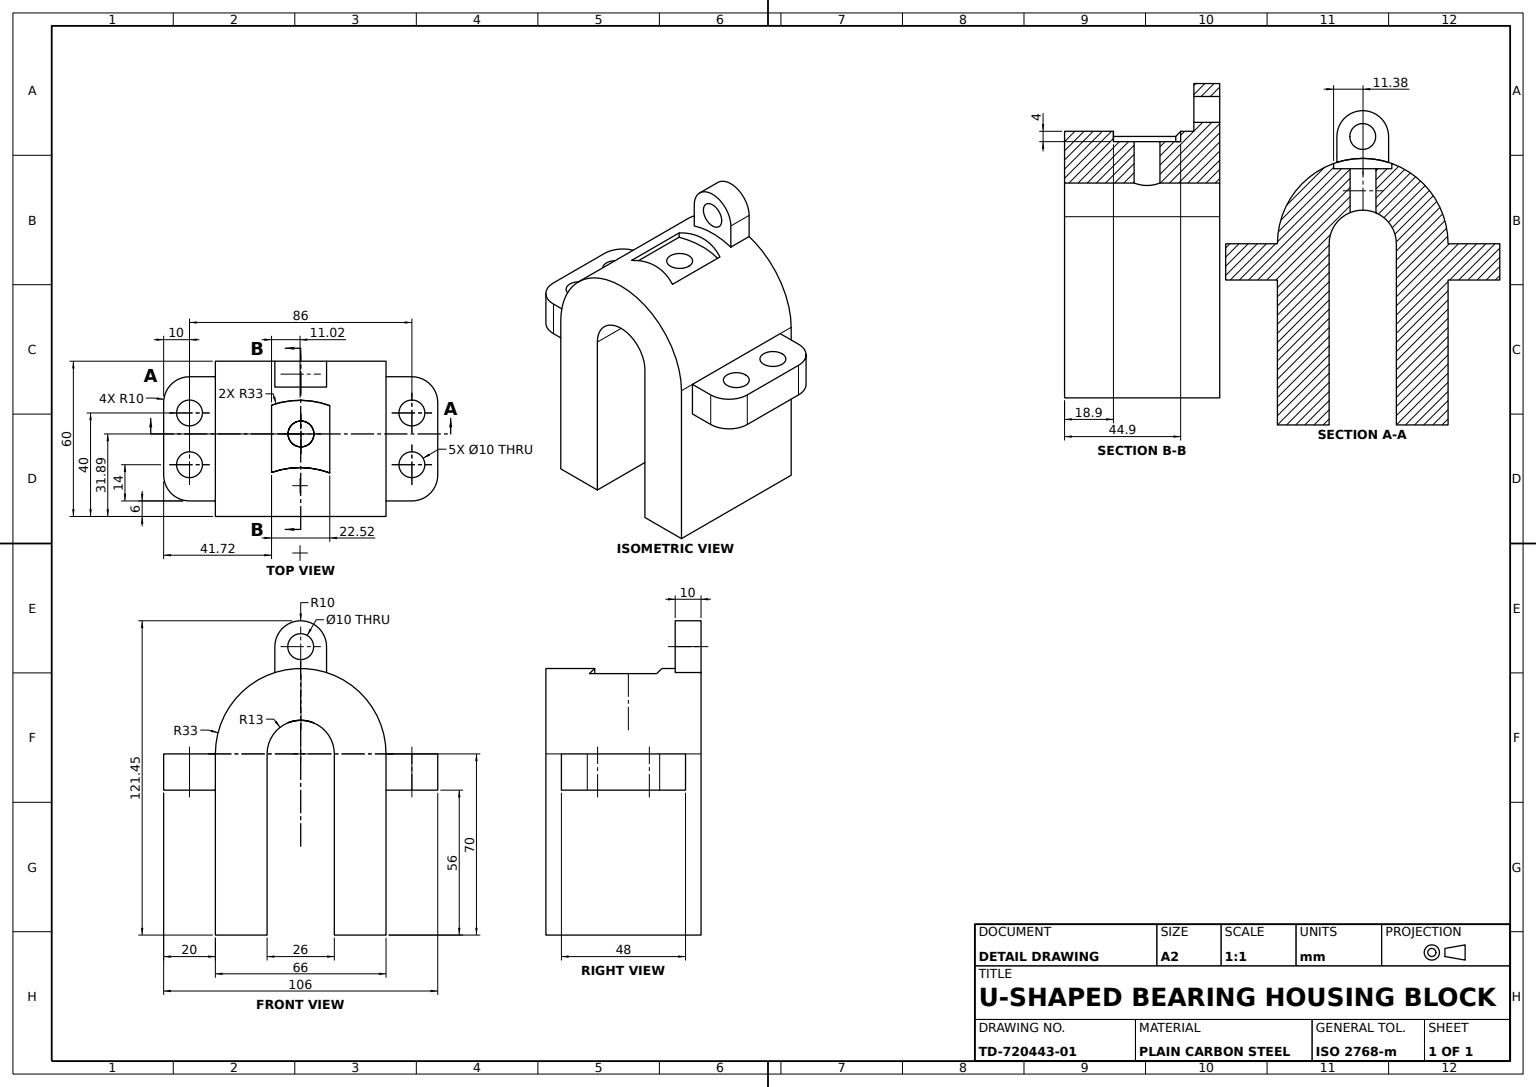
ISO-10303-21;
HEADER;
FILE_DESCRIPTION((''),'2;1');
FILE_NAME('','',(''),(''),'','','');
FILE_SCHEMA(('AUTOMOTIVE_DESIGN'));
ENDSEC;
DATA;
#1=APPLICATION_CONTEXT('');
#2=PRODUCT_CONTEXT('',#1,'mechanical');
#3=PRODUCT('','','',(#2));
#4=PRODUCT_DEFINITION_FORMATION('','',#3);
#5=PRODUCT_DEFINITION_CONTEXT('',#1,'design');
#6=PRODUCT_DEFINITION('','',#4,#5);
#7=PRODUCT_DEFINITION_SHAPE('','',#6);
#8=(LENGTH_UNIT()NAMED_UNIT(*)SI_UNIT(.MILLI.,.METRE.));
#9=(NAMED_UNIT(*)PLANE_ANGLE_UNIT()SI_UNIT($,.RADIAN.));
#10=(NAMED_UNIT(*)SI_UNIT($,.STERADIAN.)SOLID_ANGLE_UNIT());
#11=UNCERTAINTY_MEASURE_WITH_UNIT(LENGTH_MEASURE(1.E-05),#8,'distance_accuracy_value','');
#12=(GEOMETRIC_REPRESENTATION_CONTEXT(3)GLOBAL_UNCERTAINTY_ASSIGNED_CONTEXT((#11))GLOBAL_UNIT_ASSIGNED_CONTEXT((#8,#9,#10))REPRESENTATION_CONTEXT('',''));
#13=CARTESIAN_POINT('',(46.,70.,-60.));
#14=VERTEX_POINT('',#13);
#15=CARTESIAN_POINT('',(46.,0.,-60.));
#16=VERTEX_POINT('',#15);
#17=DIRECTION('',(0.,-1.,0.));
#18=VECTOR('',#17,1000.);
#19=LINE('',#13,#18);
#20=EDGE_CURVE('',#14,#16,#19,.T.);
#21=ORIENTED_EDGE('',*,*,#20,.T.);
#22=CARTESIAN_POINT('',(46.,0.,0.));
#23=VERTEX_POINT('',#22);
#24=DIRECTION('',(0.,0.,1.));
#25=VECTOR('',#24,1000.);
#26=LINE('',#15,#25);
#27=EDGE_CURVE('',#16,#23,#26,.T.);
#28=ORIENTED_EDGE('',*,*,#27,.T.);
#29=CARTESIAN_POINT('',(46.,70.,0.));
#30=VERTEX_POINT('',#29);
#31=LINE('',#29,#18);
#32=EDGE_CURVE('',#30,#23,#31,.T.);
#33=ORIENTED_EDGE('',*,*,#32,.F.);
#34=LINE('',#13,#25);
#35=EDGE_CURVE('',#14,#30,#34,.T.);
#36=ORIENTED_EDGE('',*,*,#35,.F.);
#37=EDGE_LOOP('',(#21,#28,#33,#36));
#38=FACE_OUTER_BOUND('',#37,.T.);
#39=DIRECTION('',(-1.,0.,0.));
#40=AXIS2_PLACEMENT_3D('',#13,#39,#17);
#41=PLANE('',#40);
#42=ADVANCED_FACE('',(#38),#41,.T.);
#43=CARTESIAN_POINT('',(-10.,56.,-54.));
#44=VERTEX_POINT('',#43);
#45=CARTESIAN_POINT('',(-10.,70.,-54.));
#46=VERTEX_POINT('',#45);
#47=DIRECTION('',(0.,1.,0.));
#48=VECTOR('',#47,1000.);
#49=LINE('',#43,#48);
#50=EDGE_CURVE('',#44,#46,#49,.T.);
#51=ORIENTED_EDGE('',*,*,#50,.F.);
#52=CARTESIAN_POINT('',(-20.,56.,-44.));
#53=VERTEX_POINT('',#52);
#54=CARTESIAN_POINT('',(-10.,56.,-44.));
#55=DIRECTION('',(0.,0.,-1.));
#56=AXIS2_PLACEMENT_3D('',#54,#17,#55);
#57=CIRCLE('',#56,10.);
#58=EDGE_CURVE('',#53,#44,#57,.T.);
#59=ORIENTED_EDGE('',*,*,#58,.F.);
#60=CARTESIAN_POINT('',(-20.,70.,-44.));
#61=VERTEX_POINT('',#60);
#62=LINE('',#52,#18);
#63=EDGE_CURVE('',#61,#53,#62,.T.);
#64=ORIENTED_EDGE('',*,*,#63,.F.);
#65=CARTESIAN_POINT('',(-10.,70.,-44.));
#66=AXIS2_PLACEMENT_3D('',#65,#47,#55);
#67=CIRCLE('',#66,10.);
#68=EDGE_CURVE('',#46,#61,#67,.T.);
#69=ORIENTED_EDGE('',*,*,#68,.F.);
#70=EDGE_LOOP('',(#51,#59,#64,#69));
#71=FACE_OUTER_BOUND('',#70,.T.);
#72=AXIS2_PLACEMENT_3D('',#54,#47,#24);
#73=CYLINDRICAL_SURFACE('',#72,10.);
#74=ADVANCED_FACE('',(#71),#73,.T.);
#75=CARTESIAN_POINT('',(20.,70.,-60.));
#76=VERTEX_POINT('',#75);
#77=CARTESIAN_POINT('',(33.,70.,-60.));
#78=AXIS2_PLACEMENT_3D('',#77,#55,#39);
#79=CIRCLE('',#78,13.);
#80=EDGE_CURVE('',#76,#14,#79,.T.);
#81=ORIENTED_EDGE('',*,*,#80,.F.);
#82=CARTESIAN_POINT('',(20.,0.,-60.));
#83=VERTEX_POINT('',#82);
#84=LINE('',#82,#48);
#85=EDGE_CURVE('',#83,#76,#84,.T.);
#86=ORIENTED_EDGE('',*,*,#85,.F.);
#87=CARTESIAN_POINT('',(0.,0.,-60.));
#88=VERTEX_POINT('',#87);
#89=DIRECTION('',(1.,0.,0.));
#90=VECTOR('',#89,1000.);
#91=LINE('',#87,#90);
#92=EDGE_CURVE('',#88,#83,#91,.T.);
#93=ORIENTED_EDGE('',*,*,#92,.F.);
#94=CARTESIAN_POINT('',(0.,70.,-60.));
#95=VERTEX_POINT('',#94);
#96=LINE('',#87,#18);
#97=EDGE_CURVE('',#95,#88,#96,.T.);
#98=ORIENTED_EDGE('',*,*,#97,.F.);
#99=CARTESIAN_POINT('',(23.,101.44837,-60.));
#100=VERTEX_POINT('',#99);
#101=AXIS2_PLACEMENT_3D('',#77,#24,#39);
#102=CIRCLE('',#101,33.);
#103=EDGE_CURVE('',#100,#95,#102,.T.);
#104=ORIENTED_EDGE('',*,*,#103,.F.);
#105=CARTESIAN_POINT('',(23.,111.44837,-60.));
#106=VERTEX_POINT('',#105);
#107=LINE('',#105,#48);
#108=EDGE_CURVE('',#100,#106,#107,.T.);
#109=ORIENTED_EDGE('',*,*,#108,.T.);
#110=CARTESIAN_POINT('',(43.,111.44837,-60.));
#111=VERTEX_POINT('',#110);
#112=CARTESIAN_POINT('',(33.,111.44837,-60.));
#113=AXIS2_PLACEMENT_3D('',#112,#55,#89);
#114=CIRCLE('',#113,10.);
#115=EDGE_CURVE('',#106,#111,#114,.T.);
#116=ORIENTED_EDGE('',*,*,#115,.T.);
#117=CARTESIAN_POINT('',(43.,101.44837,-60.));
#118=VERTEX_POINT('',#117);
#119=LINE('',#117,#18);
#120=EDGE_CURVE('',#111,#118,#119,.T.);
#121=ORIENTED_EDGE('',*,*,#120,.T.);
#122=CARTESIAN_POINT('',(66.,70.,-60.));
#123=VERTEX_POINT('',#122);
#124=EDGE_CURVE('',#123,#118,#102,.T.);
#125=ORIENTED_EDGE('',*,*,#124,.F.);
#126=CARTESIAN_POINT('',(66.,0.,-60.));
#127=VERTEX_POINT('',#126);
#128=LINE('',#122,#48);
#129=EDGE_CURVE('',#127,#123,#128,.T.);
#130=ORIENTED_EDGE('',*,*,#129,.F.);
#131=LINE('',#15,#90);
#132=EDGE_CURVE('',#16,#127,#131,.T.);
#133=ORIENTED_EDGE('',*,*,#132,.F.);
#134=ORIENTED_EDGE('',*,*,#20,.F.);
#135=EDGE_LOOP('',(#81,#86,#93,#98,#104,#109,#116,#121,#125,#130,#133,#134));
#136=FACE_OUTER_BOUND('',#135,.T.);
#137=CARTESIAN_POINT('',(28.,111.44837,-60.));
#138=VERTEX_POINT('',#137);
#139=CARTESIAN_POINT('',(38.,111.44837,-60.));
#140=VERTEX_POINT('',#139);
#141=AXIS2_PLACEMENT_3D('',#112,#55,#39);
#142=CIRCLE('',#141,5.);
#143=EDGE_CURVE('',#138,#140,#142,.T.);
#144=ORIENTED_EDGE('',*,*,#143,.F.);
#145=EDGE_CURVE('',#140,#138,#142,.T.);
#146=ORIENTED_EDGE('',*,*,#145,.F.);
#147=EDGE_LOOP('',(#144,#146));
#148=FACE_BOUND('',#147,.T.);
#149=PLANE('',#78);
#150=ADVANCED_FACE('',(#136,#148),#149,.T.);
#151=CARTESIAN_POINT('',(86.,70.,-44.));
#152=VERTEX_POINT('',#151);
#153=CARTESIAN_POINT('',(76.,70.,-54.));
#154=VERTEX_POINT('',#153);
#155=CARTESIAN_POINT('',(76.,70.,-44.));
#156=AXIS2_PLACEMENT_3D('',#155,#47,#24);
#157=CIRCLE('',#156,10.);
#158=EDGE_CURVE('',#152,#154,#157,.T.);
#159=ORIENTED_EDGE('',*,*,#158,.F.);
#160=CARTESIAN_POINT('',(86.,56.,-44.));
#161=VERTEX_POINT('',#160);
#162=LINE('',#160,#48);
#163=EDGE_CURVE('',#161,#152,#162,.T.);
#164=ORIENTED_EDGE('',*,*,#163,.F.);
#165=CARTESIAN_POINT('',(76.,56.,-54.));
#166=VERTEX_POINT('',#165);
#167=CARTESIAN_POINT('',(76.,56.,-44.));
#168=AXIS2_PLACEMENT_3D('',#167,#17,#24);
#169=CIRCLE('',#168,10.);
#170=EDGE_CURVE('',#166,#161,#169,.T.);
#171=ORIENTED_EDGE('',*,*,#170,.F.);
#172=LINE('',#165,#18);
#173=EDGE_CURVE('',#154,#166,#172,.T.);
#174=ORIENTED_EDGE('',*,*,#173,.F.);
#175=EDGE_LOOP('',(#159,#164,#171,#174));
#176=FACE_OUTER_BOUND('',#175,.T.);
#177=AXIS2_PLACEMENT_3D('',#167,#47,#24);
#178=CYLINDRICAL_SURFACE('',#177,10.);
#179=ADVANCED_FACE('',(#176),#178,.T.);
#180=CARTESIAN_POINT('',(44.244993,99.,-42.828348));
#181=VERTEX_POINT('',#180);
#182=CARTESIAN_POINT('',(44.244993,101.024992,-42.828348));
#183=VERTEX_POINT('',#182);
#184=LINE('',#180,#48);
#185=EDGE_CURVE('',#181,#183,#184,.T.);
#186=ORIENTED_EDGE('',*,*,#185,.F.);
#187=CARTESIAN_POINT('',(44.244993,99.,-16.828348));
#188=VERTEX_POINT('',#187);
#189=VECTOR('',#55,1000.);
#190=LINE('',#180,#189);
#191=EDGE_CURVE('',#188,#181,#190,.T.);
#192=ORIENTED_EDGE('',*,*,#191,.F.);
#193=CARTESIAN_POINT('',(44.244993,101.024992,-16.828348));
#194=VERTEX_POINT('',#193);
#195=LINE('',#187,#48);
#196=EDGE_CURVE('',#188,#194,#195,.T.);
#197=ORIENTED_EDGE('',*,*,#196,.T.);
#198=CARTESIAN_POINT('',(44.244993,101.024992,-60.));
#199=LINE('',#198,#189);
#200=EDGE_CURVE('',#194,#183,#199,.T.);
#201=ORIENTED_EDGE('',*,*,#200,.T.);
#202=EDGE_LOOP('',(#186,#192,#197,#201));
#203=FACE_OUTER_BOUND('',#202,.T.);
#204=AXIS2_PLACEMENT_3D('',#180,#89,#55);
#205=PLANE('',#204);
#206=ADVANCED_FACE('',(#203),#205,.F.);
#207=CARTESIAN_POINT('',(43.,111.44837,-50.));
#208=VERTEX_POINT('',#207);
#209=LINE('',#207,#189);
#210=EDGE_CURVE('',#208,#111,#209,.T.);
#211=ORIENTED_EDGE('',*,*,#210,.F.);
#212=CARTESIAN_POINT('',(43.,101.44837,-50.));
#213=VERTEX_POINT('',#212);
#214=LINE('',#212,#18);
#215=EDGE_CURVE('',#208,#213,#214,.T.);
#216=ORIENTED_EDGE('',*,*,#215,.T.);
#217=LINE('',#212,#189);
#218=EDGE_CURVE('',#213,#118,#217,.T.);
#219=ORIENTED_EDGE('',*,*,#218,.T.);
#220=ORIENTED_EDGE('',*,*,#120,.F.);
#221=EDGE_LOOP('',(#211,#216,#219,#220));
#222=FACE_OUTER_BOUND('',#221,.T.);
#223=AXIS2_PLACEMENT_3D('',#212,#89,#55);
#224=PLANE('',#223);
#225=ADVANCED_FACE('',(#222),#224,.T.);
#226=CARTESIAN_POINT('',(-20.,70.,-16.));
#227=VERTEX_POINT('',#226);
#228=CARTESIAN_POINT('',(-20.,70.,-54.));
#229=LINE('',#228,#25);
#230=EDGE_CURVE('',#61,#227,#229,.T.);
#231=ORIENTED_EDGE('',*,*,#230,.F.);
#232=ORIENTED_EDGE('',*,*,#63,.T.);
#233=CARTESIAN_POINT('',(-20.,56.,-16.));
#234=VERTEX_POINT('',#233);
#235=CARTESIAN_POINT('',(-20.,56.,-54.));
#236=LINE('',#235,#25);
#237=EDGE_CURVE('',#53,#234,#236,.T.);
#238=ORIENTED_EDGE('',*,*,#237,.T.);
#239=LINE('',#233,#48);
#240=EDGE_CURVE('',#234,#227,#239,.T.);
#241=ORIENTED_EDGE('',*,*,#240,.T.);
#242=EDGE_LOOP('',(#231,#232,#238,#241));
#243=FACE_OUTER_BOUND('',#242,.T.);
#244=AXIS2_PLACEMENT_3D('',#235,#39,#24);
#245=PLANE('',#244);
#246=ADVANCED_FACE('',(#243),#245,.T.);
#247=CARTESIAN_POINT('',(86.,70.,-16.));
#248=VERTEX_POINT('',#247);
#249=CARTESIAN_POINT('',(86.,56.,-16.));
#250=VERTEX_POINT('',#249);
#251=LINE('',#249,#18);
#252=EDGE_CURVE('',#248,#250,#251,.T.);
#253=ORIENTED_EDGE('',*,*,#252,.T.);
#254=CARTESIAN_POINT('',(86.,56.,-54.));
#255=LINE('',#254,#189);
#256=EDGE_CURVE('',#250,#161,#255,.T.);
#257=ORIENTED_EDGE('',*,*,#256,.T.);
#258=ORIENTED_EDGE('',*,*,#163,.T.);
#259=CARTESIAN_POINT('',(86.,70.,-54.));
#260=LINE('',#259,#189);
#261=EDGE_CURVE('',#248,#152,#260,.T.);
#262=ORIENTED_EDGE('',*,*,#261,.F.);
#263=EDGE_LOOP('',(#253,#257,#258,#262));
#264=FACE_OUTER_BOUND('',#263,.T.);
#265=AXIS2_PLACEMENT_3D('',#254,#89,#55);
#266=PLANE('',#265);
#267=ADVANCED_FACE('',(#264),#266,.T.);
#268=CARTESIAN_POINT('',(0.,56.,-54.));
#269=VERTEX_POINT('',#268);
#270=CARTESIAN_POINT('',(0.,70.,-54.));
#271=VERTEX_POINT('',#270);
#272=LINE('',#268,#48);
#273=EDGE_CURVE('',#269,#271,#272,.T.);
#274=ORIENTED_EDGE('',*,*,#273,.T.);
#275=LINE('',#94,#25);
#276=EDGE_CURVE('',#95,#271,#275,.T.);
#277=ORIENTED_EDGE('',*,*,#276,.F.);
#278=ORIENTED_EDGE('',*,*,#97,.T.);
#279=CARTESIAN_POINT('',(0.,0.,0.));
#280=VERTEX_POINT('',#279);
#281=LINE('',#87,#25);
#282=EDGE_CURVE('',#88,#280,#281,.T.);
#283=ORIENTED_EDGE('',*,*,#282,.T.);
#284=CARTESIAN_POINT('',(0.,70.,0.));
#285=VERTEX_POINT('',#284);
#286=LINE('',#279,#18);
#287=EDGE_CURVE('',#285,#280,#286,.T.);
#288=ORIENTED_EDGE('',*,*,#287,.F.);
#289=CARTESIAN_POINT('',(0.,70.,-6.));
#290=VERTEX_POINT('',#289);
#291=EDGE_CURVE('',#290,#285,#275,.T.);
#292=ORIENTED_EDGE('',*,*,#291,.F.);
#293=CARTESIAN_POINT('',(0.,56.,-6.));
#294=VERTEX_POINT('',#293);
#295=LINE('',#293,#48);
#296=EDGE_CURVE('',#294,#290,#295,.T.);
#297=ORIENTED_EDGE('',*,*,#296,.F.);
#298=LINE('',#268,#189);
#299=EDGE_CURVE('',#294,#269,#298,.T.);
#300=ORIENTED_EDGE('',*,*,#299,.T.);
#301=EDGE_LOOP('',(#274,#277,#278,#283,#288,#292,#297,#300));
#302=FACE_OUTER_BOUND('',#301,.T.);
#303=AXIS2_PLACEMENT_3D('',#87,#39,#24);
#304=PLANE('',#303);
#305=ADVANCED_FACE('',(#302),#304,.T.);
#306=CARTESIAN_POINT('',(38.,111.44837,-50.));
#307=VERTEX_POINT('',#306);
#308=CARTESIAN_POINT('',(28.,111.44837,-50.));
#309=VERTEX_POINT('',#308);
#310=CARTESIAN_POINT('',(33.,111.44837,-50.));
#311=AXIS2_PLACEMENT_3D('',#310,#55,#39);
#312=CIRCLE('',#311,5.);
#313=EDGE_CURVE('',#307,#309,#312,.T.);
#314=ORIENTED_EDGE('',*,*,#313,.F.);
#315=LINE('',#306,#189);
#316=EDGE_CURVE('',#307,#140,#315,.T.);
#317=ORIENTED_EDGE('',*,*,#316,.T.);
#318=ORIENTED_EDGE('',*,*,#145,.T.);
#319=LINE('',#308,#189);
#320=EDGE_CURVE('',#309,#138,#319,.T.);
#321=ORIENTED_EDGE('',*,*,#320,.F.);
#322=EDGE_LOOP('',(#314,#317,#318,#321));
#323=FACE_OUTER_BOUND('',#322,.T.);
#324=CYLINDRICAL_SURFACE('',#311,5.);
#325=ADVANCED_FACE('',(#323),#324,.F.);
#326=CARTESIAN_POINT('',(76.,70.,-25.));
#327=VERTEX_POINT('',#326);
#328=CARTESIAN_POINT('',(76.,70.,-15.));
#329=VERTEX_POINT('',#328);
#330=CARTESIAN_POINT('',(76.,70.,-20.));
#331=AXIS2_PLACEMENT_3D('',#330,#47,#24);
#332=CIRCLE('',#331,5.);
#333=EDGE_CURVE('',#327,#329,#332,.T.);
#334=ORIENTED_EDGE('',*,*,#333,.T.);
#335=CARTESIAN_POINT('',(76.,56.,-15.));
#336=VERTEX_POINT('',#335);
#337=LINE('',#335,#48);
#338=EDGE_CURVE('',#336,#329,#337,.T.);
#339=ORIENTED_EDGE('',*,*,#338,.F.);
#340=CARTESIAN_POINT('',(76.,56.,-25.));
#341=VERTEX_POINT('',#340);
#342=CARTESIAN_POINT('',(76.,56.,-20.));
#343=AXIS2_PLACEMENT_3D('',#342,#47,#24);
#344=CIRCLE('',#343,5.);
#345=EDGE_CURVE('',#341,#336,#344,.T.);
#346=ORIENTED_EDGE('',*,*,#345,.F.);
#347=LINE('',#340,#48);
#348=EDGE_CURVE('',#341,#327,#347,.T.);
#349=ORIENTED_EDGE('',*,*,#348,.T.);
#350=EDGE_LOOP('',(#334,#339,#346,#349));
#351=FACE_OUTER_BOUND('',#350,.T.);
#352=CYLINDRICAL_SURFACE('',#343,5.);
#353=ADVANCED_FACE('',(#351),#352,.F.);
#354=CARTESIAN_POINT('',(66.,56.,-54.));
#355=VERTEX_POINT('',#354);
#356=VECTOR('',#39,1000.);
#357=LINE('',#354,#356);
#358=EDGE_CURVE('',#166,#355,#357,.T.);
#359=ORIENTED_EDGE('',*,*,#358,.T.);
#360=CARTESIAN_POINT('',(66.,70.,-54.));
#361=VERTEX_POINT('',#360);
#362=LINE('',#354,#48);
#363=EDGE_CURVE('',#355,#361,#362,.T.);
#364=ORIENTED_EDGE('',*,*,#363,.T.);
#365=LINE('',#360,#356);
#366=EDGE_CURVE('',#154,#361,#365,.T.);
#367=ORIENTED_EDGE('',*,*,#366,.F.);
#368=ORIENTED_EDGE('',*,*,#173,.T.);
#369=EDGE_LOOP('',(#359,#364,#367,#368));
#370=FACE_OUTER_BOUND('',#369,.T.);
#371=AXIS2_PLACEMENT_3D('',#354,#55,#39);
#372=PLANE('',#371);
#373=ADVANCED_FACE('',(#370),#372,.T.);
#374=CARTESIAN_POINT('',(23.,111.44837,-50.));
#375=VERTEX_POINT('',#374);
#376=LINE('',#374,#189);
#377=EDGE_CURVE('',#375,#106,#376,.T.);
#378=ORIENTED_EDGE('',*,*,#377,.F.);
#379=AXIS2_PLACEMENT_3D('',#310,#55,#89);
#380=CIRCLE('',#379,10.);
#381=EDGE_CURVE('',#375,#208,#380,.T.);
#382=ORIENTED_EDGE('',*,*,#381,.T.);
#383=ORIENTED_EDGE('',*,*,#210,.T.);
#384=ORIENTED_EDGE('',*,*,#115,.F.);
#385=EDGE_LOOP('',(#378,#382,#383,#384));
#386=FACE_OUTER_BOUND('',#385,.T.);
#387=CYLINDRICAL_SURFACE('',#311,10.);
#388=ADVANCED_FACE('',(#386),#387,.T.);
#389=CARTESIAN_POINT('',(-10.,56.,-35.));
#390=VERTEX_POINT('',#389);
#391=CARTESIAN_POINT('',(-10.,70.,-35.));
#392=VERTEX_POINT('',#391);
#393=LINE('',#389,#48);
#394=EDGE_CURVE('',#390,#392,#393,.T.);
#395=ORIENTED_EDGE('',*,*,#394,.T.);
#396=CARTESIAN_POINT('',(-10.,70.,-45.));
#397=VERTEX_POINT('',#396);
#398=CARTESIAN_POINT('',(-10.,70.,-40.));
#399=AXIS2_PLACEMENT_3D('',#398,#47,#55);
#400=CIRCLE('',#399,5.);
#401=EDGE_CURVE('',#392,#397,#400,.T.);
#402=ORIENTED_EDGE('',*,*,#401,.T.);
#403=CARTESIAN_POINT('',(-10.,56.,-45.));
#404=VERTEX_POINT('',#403);
#405=LINE('',#403,#48);
#406=EDGE_CURVE('',#404,#397,#405,.T.);
#407=ORIENTED_EDGE('',*,*,#406,.F.);
#408=CARTESIAN_POINT('',(-10.,56.,-40.));
#409=AXIS2_PLACEMENT_3D('',#408,#47,#55);
#410=CIRCLE('',#409,5.);
#411=EDGE_CURVE('',#390,#404,#410,.T.);
#412=ORIENTED_EDGE('',*,*,#411,.F.);
#413=EDGE_LOOP('',(#395,#402,#407,#412));
#414=FACE_OUTER_BOUND('',#413,.T.);
#415=AXIS2_PLACEMENT_3D('',#408,#47,#24);
#416=CYLINDRICAL_SURFACE('',#415,5.);
#417=ADVANCED_FACE('',(#414),#416,.F.);
#418=CARTESIAN_POINT('',(21.724815,99.,-43.));
#419=VERTEX_POINT('',#418);
#420=CARTESIAN_POINT('',(32.748476,99.,-11.895677));
#421=AXIS2_PLACEMENT_3D('',#420,#47,#89);
#422=CIRCLE('',#421,33.);
#423=EDGE_CURVE('',#181,#419,#422,.T.);
#424=ORIENTED_EDGE('',*,*,#423,.F.);
#425=ORIENTED_EDGE('',*,*,#185,.T.);
#426=CARTESIAN_POINT('',(21.724815,101.014032,-43.));
#427=VERTEX_POINT('',#426);
#428=CARTESIAN_POINT('',(42.498921,101.657855,-43.477298));
#429=CARTESIAN_POINT('',(40.686339,102.149464,-43.984127));
#430=CARTESIAN_POINT('',(38.329664,102.570292,-44.423823));
#431=CARTESIAN_POINT('',(37.853746,102.644698,-44.501994));
#432=CARTESIAN_POINT('',(36.892391,102.773228,-44.63806));
#433=CARTESIAN_POINT('',(36.405223,102.827472,-44.696089));
#434=CARTESIAN_POINT('',(34.945985,102.957048,-44.836931));
#435=CARTESIAN_POINT('',(33.974512,102.999871,-44.887162));
#436=CARTESIAN_POINT('',(32.034218,103.000128,-44.902208));
#437=CARTESIAN_POINT('',(31.065396,102.957558,-44.867019));
#438=CARTESIAN_POINT('',(29.614157,102.829437,-44.750077));
#439=CARTESIAN_POINT('',(29.130743,102.776003,-44.700388));
#440=CARTESIAN_POINT('',(28.164588,102.647455,-44.579389));
#441=CARTESIAN_POINT('',(27.682559,102.572354,-44.508087));
#442=CARTESIAN_POINT('',(25.304489,102.148305,-44.102997));
#443=CARTESIAN_POINT('',(23.479701,101.652023,-43.621948));
#444=B_SPLINE_CURVE_WITH_KNOTS('',3,(#182,#428,#429,#430,#431,#432,#433,#434,#435,#436,#437,#438,#439,#440,#441,#442,#443,#426),.UNSPECIFIED.,.F.,.F.,(4,2,2,2,2,2,2,2,4),(0.,0.005828181,0.007285226,0.008742271,0.011656362,0.014570452,0.016027497,0.017484543,0.023312723),.UNSPECIFIED.);
#445=EDGE_CURVE('',#183,#427,#444,.T.);
#446=ORIENTED_EDGE('',*,*,#445,.T.);
#447=LINE('',#418,#48);
#448=EDGE_CURVE('',#419,#427,#447,.T.);
#449=ORIENTED_EDGE('',*,*,#448,.F.);
#450=EDGE_LOOP('',(#424,#425,#446,#449));
#451=FACE_OUTER_BOUND('',#450,.T.);
#452=AXIS2_PLACEMENT_3D('',#420,#47,#39);
#453=CYLINDRICAL_SURFACE('',#452,33.);
#454=ADVANCED_FACE('',(#451),#453,.F.);
#455=LINE('',#122,#25);
#456=EDGE_CURVE('',#123,#361,#455,.T.);
#457=ORIENTED_EDGE('',*,*,#456,.F.);
#458=ORIENTED_EDGE('',*,*,#124,.T.);
#459=ORIENTED_EDGE('',*,*,#218,.F.);
#460=CARTESIAN_POINT('',(23.,101.44837,-50.));
#461=VERTEX_POINT('',#460);
#462=CARTESIAN_POINT('',(33.,70.,-50.));
#463=AXIS2_PLACEMENT_3D('',#462,#24,#89);
#464=CIRCLE('',#463,33.);
#465=EDGE_CURVE('',#213,#461,#464,.T.);
#466=ORIENTED_EDGE('',*,*,#465,.T.);
#467=LINE('',#460,#189);
#468=EDGE_CURVE('',#461,#100,#467,.T.);
#469=ORIENTED_EDGE('',*,*,#468,.T.);
#470=ORIENTED_EDGE('',*,*,#103,.T.);
#471=ORIENTED_EDGE('',*,*,#276,.T.);
#472=LINE('',#270,#189);
#473=EDGE_CURVE('',#290,#271,#472,.T.);
#474=ORIENTED_EDGE('',*,*,#473,.F.);
#475=ORIENTED_EDGE('',*,*,#291,.T.);
#476=CARTESIAN_POINT('',(66.,70.,0.));
#477=VERTEX_POINT('',#476);
#478=CARTESIAN_POINT('',(33.,70.,0.));
#479=AXIS2_PLACEMENT_3D('',#478,#24,#39);
#480=CIRCLE('',#479,33.);
#481=EDGE_CURVE('',#477,#285,#480,.T.);
#482=ORIENTED_EDGE('',*,*,#481,.F.);
#483=CARTESIAN_POINT('',(66.,70.,-6.));
#484=VERTEX_POINT('',#483);
#485=EDGE_CURVE('',#484,#477,#455,.T.);
#486=ORIENTED_EDGE('',*,*,#485,.F.);
#487=LINE('',#360,#25);
#488=EDGE_CURVE('',#361,#484,#487,.T.);
#489=ORIENTED_EDGE('',*,*,#488,.F.);
#490=EDGE_LOOP('',(#457,#458,#459,#466,#469,#470,#471,#474,#475,#482,#486,#489));
#491=FACE_OUTER_BOUND('',#490,.T.);
#492=CARTESIAN_POINT('',(21.724815,101.014032,-17.));
#493=VERTEX_POINT('',#492);
#494=CARTESIAN_POINT('',(21.724815,101.014032,-60.));
#495=LINE('',#494,#25);
#496=EDGE_CURVE('',#427,#493,#495,.T.);
#497=ORIENTED_EDGE('',*,*,#496,.F.);
#498=ORIENTED_EDGE('',*,*,#445,.F.);
#499=ORIENTED_EDGE('',*,*,#200,.F.);
#500=CARTESIAN_POINT('',(23.47909,101.651801,-17.621731));
#501=CARTESIAN_POINT('',(25.298362,102.146103,-18.100848));
#502=CARTESIAN_POINT('',(27.661107,102.568799,-18.504702));
#503=CARTESIAN_POINT('',(28.138124,102.643503,-18.575646));
#504=CARTESIAN_POINT('',(29.101428,102.772508,-18.697121));
#505=CARTESIAN_POINT('',(29.589441,102.826927,-18.747759));
#506=CARTESIAN_POINT('',(31.050515,102.956878,-18.866452));
#507=CARTESIAN_POINT('',(32.022609,102.999787,-18.901956));
#508=CARTESIAN_POINT('',(33.962971,103.000211,-18.88759));
#509=CARTESIAN_POINT('',(34.93124,102.957722,-18.837717));
#510=CARTESIAN_POINT('',(36.380771,102.829951,-18.698757));
#511=CARTESIAN_POINT('',(36.863469,102.776672,-18.64173));
#512=CARTESIAN_POINT('',(37.827897,102.648553,-18.506053));
#513=CARTESIAN_POINT('',(38.308703,102.573759,-18.427457));
#514=CARTESIAN_POINT('',(40.68037,102.151607,-17.986322));
#515=CARTESIAN_POINT('',(42.498324,101.658071,-17.477519));
#516=B_SPLINE_CURVE_WITH_KNOTS('',3,(#492,#500,#501,#502,#503,#504,#505,#506,#507,#508,#509,#510,#511,#512,#513,#514,#515,#193),.UNSPECIFIED.,.F.,.F.,(4,2,2,2,2,2,2,2,4),(0.,0.005827939,0.007284924,0.008741909,0.011655878,0.014569848,0.016026833,0.017483818,0.023311757),.UNSPECIFIED.);
#517=EDGE_CURVE('',#493,#194,#516,.T.);
#518=ORIENTED_EDGE('',*,*,#517,.F.);
#519=EDGE_LOOP('',(#497,#498,#499,#518));
#520=FACE_BOUND('',#519,.T.);
#521=AXIS2_PLACEMENT_3D('',#77,#24,#89);
#522=CYLINDRICAL_SURFACE('',#521,33.);
#523=ADVANCED_FACE('',(#491,#520),#522,.T.);
#524=ORIENTED_EDGE('',*,*,#240,.F.);
#525=CARTESIAN_POINT('',(-10.,56.,-6.));
#526=VERTEX_POINT('',#525);
#527=CARTESIAN_POINT('',(-10.,56.,-16.));
#528=AXIS2_PLACEMENT_3D('',#527,#17,#55);
#529=CIRCLE('',#528,10.);
#530=EDGE_CURVE('',#526,#234,#529,.T.);
#531=ORIENTED_EDGE('',*,*,#530,.F.);
#532=CARTESIAN_POINT('',(-10.,70.,-6.));
#533=VERTEX_POINT('',#532);
#534=LINE('',#525,#18);
#535=EDGE_CURVE('',#533,#526,#534,.T.);
#536=ORIENTED_EDGE('',*,*,#535,.F.);
#537=CARTESIAN_POINT('',(-10.,70.,-16.));
#538=AXIS2_PLACEMENT_3D('',#537,#47,#55);
#539=CIRCLE('',#538,10.);
#540=EDGE_CURVE('',#227,#533,#539,.T.);
#541=ORIENTED_EDGE('',*,*,#540,.F.);
#542=EDGE_LOOP('',(#524,#531,#536,#541));
#543=FACE_OUTER_BOUND('',#542,.T.);
#544=CYLINDRICAL_SURFACE('',#528,10.);
#545=ADVANCED_FACE('',(#543),#544,.T.);
#546=ORIENTED_EDGE('',*,*,#338,.T.);
#547=EDGE_CURVE('',#329,#327,#332,.T.);
#548=ORIENTED_EDGE('',*,*,#547,.T.);
#549=ORIENTED_EDGE('',*,*,#348,.F.);
#550=EDGE_CURVE('',#336,#341,#344,.T.);
#551=ORIENTED_EDGE('',*,*,#550,.F.);
#552=EDGE_LOOP('',(#546,#548,#549,#551));
#553=FACE_OUTER_BOUND('',#552,.T.);
#554=ADVANCED_FACE('',(#553),#352,.F.);
#555=ORIENTED_EDGE('',*,*,#158,.T.);
#556=ORIENTED_EDGE('',*,*,#366,.T.);
#557=ORIENTED_EDGE('',*,*,#488,.T.);
#558=CARTESIAN_POINT('',(76.,70.,-6.));
#559=VERTEX_POINT('',#558);
#560=LINE('',#483,#90);
#561=EDGE_CURVE('',#484,#559,#560,.T.);
#562=ORIENTED_EDGE('',*,*,#561,.T.);
#563=CARTESIAN_POINT('',(76.,70.,-16.));
#564=AXIS2_PLACEMENT_3D('',#563,#47,#24);
#565=CIRCLE('',#564,10.);
#566=EDGE_CURVE('',#559,#248,#565,.T.);
#567=ORIENTED_EDGE('',*,*,#566,.T.);
#568=ORIENTED_EDGE('',*,*,#261,.T.);
#569=EDGE_LOOP('',(#555,#556,#557,#562,#567,#568));
#570=FACE_OUTER_BOUND('',#569,.T.);
#571=CARTESIAN_POINT('',(76.,70.,-35.));
#572=VERTEX_POINT('',#571);
#573=CARTESIAN_POINT('',(76.,70.,-45.));
#574=VERTEX_POINT('',#573);
#575=CARTESIAN_POINT('',(76.,70.,-40.));
#576=AXIS2_PLACEMENT_3D('',#575,#47,#24);
#577=CIRCLE('',#576,5.);
#578=EDGE_CURVE('',#572,#574,#577,.T.);
#579=ORIENTED_EDGE('',*,*,#578,.F.);
#580=EDGE_CURVE('',#574,#572,#577,.T.);
#581=ORIENTED_EDGE('',*,*,#580,.F.);
#582=EDGE_LOOP('',(#579,#581));
#583=FACE_BOUND('',#582,.T.);
#584=ORIENTED_EDGE('',*,*,#547,.F.);
#585=ORIENTED_EDGE('',*,*,#333,.F.);
#586=EDGE_LOOP('',(#584,#585));
#587=FACE_BOUND('',#586,.T.);
#588=AXIS2_PLACEMENT_3D('',#284,#47,#24);
#589=PLANE('',#588);
#590=ADVANCED_FACE('',(#570,#583,#587),#589,.T.);
#591=EDGE_CURVE('',#309,#307,#312,.T.);
#592=ORIENTED_EDGE('',*,*,#591,.F.);
#593=ORIENTED_EDGE('',*,*,#320,.T.);
#594=ORIENTED_EDGE('',*,*,#143,.T.);
#595=ORIENTED_EDGE('',*,*,#316,.F.);
#596=EDGE_LOOP('',(#592,#593,#594,#595));
#597=FACE_OUTER_BOUND('',#596,.T.);
#598=ADVANCED_FACE('',(#597),#324,.F.);
#599=CARTESIAN_POINT('',(76.,56.,-35.));
#600=VERTEX_POINT('',#599);
#601=CARTESIAN_POINT('',(76.,56.,-45.));
#602=VERTEX_POINT('',#601);
#603=CARTESIAN_POINT('',(76.,56.,-40.));
#604=AXIS2_PLACEMENT_3D('',#603,#47,#24);
#605=CIRCLE('',#604,5.);
#606=EDGE_CURVE('',#600,#602,#605,.T.);
#607=ORIENTED_EDGE('',*,*,#606,.T.);
#608=EDGE_CURVE('',#602,#600,#605,.T.);
#609=ORIENTED_EDGE('',*,*,#608,.T.);
#610=EDGE_LOOP('',(#607,#609));
#611=FACE_BOUND('',#610,.T.);
#612=ORIENTED_EDGE('',*,*,#345,.T.);
#613=ORIENTED_EDGE('',*,*,#550,.T.);
#614=EDGE_LOOP('',(#612,#613));
#615=FACE_BOUND('',#614,.T.);
#616=ORIENTED_EDGE('',*,*,#358,.F.);
#617=ORIENTED_EDGE('',*,*,#170,.T.);
#618=ORIENTED_EDGE('',*,*,#256,.F.);
#619=CARTESIAN_POINT('',(76.,56.,-6.));
#620=VERTEX_POINT('',#619);
#621=CARTESIAN_POINT('',(76.,56.,-16.));
#622=AXIS2_PLACEMENT_3D('',#621,#17,#24);
#623=CIRCLE('',#622,10.);
#624=EDGE_CURVE('',#250,#620,#623,.T.);
#625=ORIENTED_EDGE('',*,*,#624,.T.);
#626=CARTESIAN_POINT('',(66.,56.,-6.));
#627=VERTEX_POINT('',#626);
#628=LINE('',#626,#90);
#629=EDGE_CURVE('',#627,#620,#628,.T.);
#630=ORIENTED_EDGE('',*,*,#629,.F.);
#631=LINE('',#354,#25);
#632=EDGE_CURVE('',#355,#627,#631,.T.);
#633=ORIENTED_EDGE('',*,*,#632,.F.);
#634=EDGE_LOOP('',(#616,#617,#618,#625,#630,#633));
#635=FACE_OUTER_BOUND('',#634,.T.);
#636=CARTESIAN_POINT('',(0.,56.,0.));
#637=AXIS2_PLACEMENT_3D('',#636,#47,#24);
#638=PLANE('',#637);
#639=ADVANCED_FACE('',(#611,#615,#635),#638,.F.);
#640=CARTESIAN_POINT('',(66.,0.,0.));
#641=VERTEX_POINT('',#640);
#642=LINE('',#126,#25);
#643=EDGE_CURVE('',#127,#641,#642,.T.);
#644=ORIENTED_EDGE('',*,*,#643,.T.);
#645=LINE('',#22,#90);
#646=EDGE_CURVE('',#23,#641,#645,.T.);
#647=ORIENTED_EDGE('',*,*,#646,.F.);
#648=ORIENTED_EDGE('',*,*,#27,.F.);
#649=ORIENTED_EDGE('',*,*,#132,.T.);
#650=EDGE_LOOP('',(#644,#647,#648,#649));
#651=FACE_OUTER_BOUND('',#650,.T.);
#652=AXIS2_PLACEMENT_3D('',#15,#17,#55);
#653=PLANE('',#652);
#654=ADVANCED_FACE('',(#651),#653,.T.);
#655=ORIENTED_EDGE('',*,*,#80,.T.);
#656=ORIENTED_EDGE('',*,*,#35,.T.);
#657=CARTESIAN_POINT('',(20.,70.,0.));
#658=VERTEX_POINT('',#657);
#659=AXIS2_PLACEMENT_3D('',#478,#55,#39);
#660=CIRCLE('',#659,13.);
#661=EDGE_CURVE('',#658,#30,#660,.T.);
#662=ORIENTED_EDGE('',*,*,#661,.F.);
#663=LINE('',#75,#25);
#664=EDGE_CURVE('',#76,#658,#663,.T.);
#665=ORIENTED_EDGE('',*,*,#664,.F.);
#666=EDGE_LOOP('',(#655,#656,#662,#665));
#667=FACE_OUTER_BOUND('',#666,.T.);
#668=CARTESIAN_POINT('',(28.108871,82.044785,-31.89243));
#669=VERTEX_POINT('',#668);
#670=CARTESIAN_POINT('',(38.108871,81.954055,-31.89243));
#671=VERTEX_POINT('',#670);
#672=CARTESIAN_POINT('',(28.108871,82.044785,-32.226307));
#673=CARTESIAN_POINT('',(28.14197,82.058373,-32.553918));
#674=CARTESIAN_POINT('',(28.271016,82.109564,-33.197355));
#675=CARTESIAN_POINT('',(28.36869,82.1478,-33.516565));
#676=CARTESIAN_POINT('',(28.620863,82.240965,-34.120639));
#677=CARTESIAN_POINT('',(28.774715,82.295668,-34.406649));
#678=CARTESIAN_POINT('',(29.137739,82.414484,-34.947969));
#679=CARTESIAN_POINT('',(29.346632,82.478345,-35.201511));
#680=CARTESIAN_POINT('',(29.803968,82.603236,-35.65834));
#681=CARTESIAN_POINT('',(30.054732,82.665034,-35.864831));
#682=CARTESIAN_POINT('',(30.600257,82.779629,-36.230009));
#683=CARTESIAN_POINT('',(30.887058,82.830736,-36.383503));
#684=CARTESIAN_POINT('',(31.338351,82.894262,-36.571298));
#685=CARTESIAN_POINT('',(31.492322,82.913251,-36.626767));
#686=CARTESIAN_POINT('',(31.807664,82.946176,-36.722962));
#687=CARTESIAN_POINT('',(31.969699,82.960124,-36.763729));
#688=CARTESIAN_POINT('',(32.455563,82.992651,-36.860556));
#689=CARTESIAN_POINT('',(32.782489,83.002368,-36.892664));
#690=CARTESIAN_POINT('',(33.442386,82.99666,-36.892193));
#691=CARTESIAN_POINT('',(33.776978,82.980781,-36.858463));
#692=CARTESIAN_POINT('',(34.420794,82.926164,-36.728411));
#693=CARTESIAN_POINT('',(34.734017,82.887524,-36.632461));
#694=CARTESIAN_POINT('',(35.343151,82.790807,-36.377627));
#695=CARTESIAN_POINT('',(35.629252,82.734327,-36.222856));
#696=CARTESIAN_POINT('',(36.16689,82.611378,-35.861489));
#697=CARTESIAN_POINT('',(36.42071,82.54414,-35.652282));
#698=CARTESIAN_POINT('',(36.877819,82.410448,-35.193913));
#699=CARTESIAN_POINT('',(37.082305,82.343879,-34.944838));
#700=CARTESIAN_POINT('',(37.44363,82.218458,-34.405444));
#701=CARTESIAN_POINT('',(37.599943,82.159709,-34.11414));
#702=CARTESIAN_POINT('',(37.849864,82.062206,-33.513761));
#703=CARTESIAN_POINT('',(37.94576,82.022664,-33.20174));
#704=CARTESIAN_POINT('',(38.07624,81.968157,-32.552007));
#705=CARTESIAN_POINT('',(38.108871,81.954055,-32.221138));
#706=B_SPLINE_CURVE_WITH_KNOTS('',3,(#668,#672,#673,#674,#675,#676,#677,#678,#679,#680,#681,#682,#683,#684,#685,#686,#687,#688,#689,#690,#691,#692,#693,#694,#695,#696,#697,#698,#699,#700,#701,#702,#703,#704,#705,#670),.UNSPECIFIED.,.F.,.F.,(4,2,2,2,2,2,2,2,2,2,2,2,2,2,2,2,2,4),(0.,0.00098661,0.001973221,0.002959831,0.003946442,0.004933052,0.005919662,0.006412968,0.006906273,0.007892883,0.008879494,0.009866104,0.010852714,0.011839325,0.012825935,0.013812545,0.014799156,0.015785766),.UNSPECIFIED.);
#707=EDGE_CURVE('',#669,#671,#706,.T.);
#708=ORIENTED_EDGE('',*,*,#707,.F.);
#709=CARTESIAN_POINT('',(38.108871,81.954055,-31.728114));
#710=CARTESIAN_POINT('',(38.100791,81.957518,-31.563706));
#711=CARTESIAN_POINT('',(38.068177,81.971378,-31.234704));
#712=CARTESIAN_POINT('',(38.043406,81.981874,-31.069214));
#713=CARTESIAN_POINT('',(37.945697,82.02269,-30.583083));
#714=CARTESIAN_POINT('',(37.849759,82.062259,-30.270405));
#715=CARTESIAN_POINT('',(37.598036,82.160441,-29.666584));
#716=CARTESIAN_POINT('',(37.441338,82.219286,-29.37559));
#717=CARTESIAN_POINT('',(37.080705,82.344402,-28.838043));
#718=CARTESIAN_POINT('',(36.875319,82.411274,-28.587821));
#719=CARTESIAN_POINT('',(36.413644,82.54611,-28.126126));
#720=CARTESIAN_POINT('',(36.164008,82.612091,-27.921208));
#721=CARTESIAN_POINT('',(35.761462,82.704065,-27.650983));
#722=CARTESIAN_POINT('',(35.622563,82.733563,-27.567151));
#723=CARTESIAN_POINT('',(35.334902,82.789437,-27.412311));
#724=CARTESIAN_POINT('',(35.18553,82.815883,-27.341134));
#725=CARTESIAN_POINT('',(34.732187,82.887714,-27.151956));
#726=CARTESIAN_POINT('',(34.420275,82.92622,-27.056313));
#727=CARTESIAN_POINT('',(33.776571,82.980804,-26.926346));
#728=CARTESIAN_POINT('',(33.441643,82.996675,-26.892643));
#729=CARTESIAN_POINT('',(32.782529,83.002358,-26.892219));
#730=CARTESIAN_POINT('',(32.455056,82.992666,-26.924271));
#731=CARTESIAN_POINT('',(31.804348,82.949006,-27.054218));
#732=CARTESIAN_POINT('',(31.487636,82.915322,-27.151295));
#733=CARTESIAN_POINT('',(30.884398,82.830316,-27.40261));
#734=CARTESIAN_POINT('',(30.592749,82.778176,-27.55935));
#735=CARTESIAN_POINT('',(30.050978,82.664119,-27.923079));
#736=CARTESIAN_POINT('',(29.80118,82.602546,-28.12884));
#737=CARTESIAN_POINT('',(29.342203,82.477064,-28.588244));
#738=CARTESIAN_POINT('',(29.133167,82.413038,-28.843054));
#739=CARTESIAN_POINT('',(28.772966,82.295044,-29.381485));
#740=CARTESIAN_POINT('',(28.619158,82.24036,-29.667381));
#741=CARTESIAN_POINT('',(28.36619,82.146851,-30.275228));
#742=CARTESIAN_POINT('',(28.270167,82.109229,-30.591052));
#743=CARTESIAN_POINT('',(28.142002,82.058383,-31.231478));
#744=CARTESIAN_POINT('',(28.108871,82.044785,-31.558631));
#745=B_SPLINE_CURVE_WITH_KNOTS('',3,(#670,#709,#710,#711,#712,#713,#714,#715,#716,#717,#718,#719,#720,#721,#722,#723,#724,#725,#726,#727,#728,#729,#730,#731,#732,#733,#734,#735,#736,#737,#738,#739,#740,#741,#742,#743,#744,#668),.UNSPECIFIED.,.F.,.F.,(4,2,2,2,2,2,2,2,2,2,2,2,2,2,2,2,2,2,4),(0.015785766,0.016278957,0.016772147,0.017758527,0.018744908,0.019731288,0.020717669,0.021210859,0.021704049,0.02269043,0.02367681,0.024663191,0.025649571,0.026635952,0.027622332,0.028608713,0.029595093,0.030581473,0.031567854),.UNSPECIFIED.);
#746=EDGE_CURVE('',#671,#669,#745,.T.);
#747=ORIENTED_EDGE('',*,*,#746,.F.);
#748=EDGE_LOOP('',(#708,#747));
#749=FACE_BOUND('',#748,.T.);
#750=CYLINDRICAL_SURFACE('',#521,13.);
#751=ADVANCED_FACE('',(#667,#749),#750,.F.);
#752=ORIENTED_EDGE('',*,*,#578,.T.);
#753=LINE('',#601,#48);
#754=EDGE_CURVE('',#602,#574,#753,.T.);
#755=ORIENTED_EDGE('',*,*,#754,.F.);
#756=ORIENTED_EDGE('',*,*,#606,.F.);
#757=LINE('',#599,#48);
#758=EDGE_CURVE('',#600,#572,#757,.T.);
#759=ORIENTED_EDGE('',*,*,#758,.T.);
#760=EDGE_LOOP('',(#752,#755,#756,#759));
#761=FACE_OUTER_BOUND('',#760,.T.);
#762=CYLINDRICAL_SURFACE('',#604,5.);
#763=ADVANCED_FACE('',(#761),#762,.F.);
#764=ORIENTED_EDGE('',*,*,#629,.T.);
#765=LINE('',#619,#48);
#766=EDGE_CURVE('',#620,#559,#765,.T.);
#767=ORIENTED_EDGE('',*,*,#766,.T.);
#768=ORIENTED_EDGE('',*,*,#561,.F.);
#769=LINE('',#626,#48);
#770=EDGE_CURVE('',#627,#484,#769,.T.);
#771=ORIENTED_EDGE('',*,*,#770,.F.);
#772=EDGE_LOOP('',(#764,#767,#768,#771));
#773=FACE_OUTER_BOUND('',#772,.T.);
#774=AXIS2_PLACEMENT_3D('',#626,#24,#89);
#775=PLANE('',#774);
#776=ADVANCED_FACE('',(#773),#775,.T.);
#777=LINE('',#293,#90);
#778=EDGE_CURVE('',#526,#294,#777,.T.);
#779=ORIENTED_EDGE('',*,*,#778,.F.);
#780=ORIENTED_EDGE('',*,*,#530,.T.);
#781=ORIENTED_EDGE('',*,*,#237,.F.);
#782=ORIENTED_EDGE('',*,*,#58,.T.);
#783=LINE('',#268,#356);
#784=EDGE_CURVE('',#269,#44,#783,.T.);
#785=ORIENTED_EDGE('',*,*,#784,.F.);
#786=ORIENTED_EDGE('',*,*,#299,.F.);
#787=EDGE_LOOP('',(#779,#780,#781,#782,#785,#786));
#788=FACE_OUTER_BOUND('',#787,.T.);
#789=CARTESIAN_POINT('',(-10.,56.,-15.));
#790=VERTEX_POINT('',#789);
#791=CARTESIAN_POINT('',(-10.,56.,-25.));
#792=VERTEX_POINT('',#791);
#793=CARTESIAN_POINT('',(-10.,56.,-20.));
#794=AXIS2_PLACEMENT_3D('',#793,#47,#55);
#795=CIRCLE('',#794,5.);
#796=EDGE_CURVE('',#790,#792,#795,.T.);
#797=ORIENTED_EDGE('',*,*,#796,.T.);
#798=EDGE_CURVE('',#792,#790,#795,.T.);
#799=ORIENTED_EDGE('',*,*,#798,.T.);
#800=EDGE_LOOP('',(#797,#799));
#801=FACE_BOUND('',#800,.T.);
#802=EDGE_CURVE('',#404,#390,#410,.T.);
#803=ORIENTED_EDGE('',*,*,#802,.T.);
#804=ORIENTED_EDGE('',*,*,#411,.T.);
#805=EDGE_LOOP('',(#803,#804));
#806=FACE_BOUND('',#805,.T.);
#807=AXIS2_PLACEMENT_3D('',#636,#17,#55);
#808=PLANE('',#807);
#809=ADVANCED_FACE('',(#788,#801,#806),#808,.T.);
#810=LINE('',#476,#48);
#811=EDGE_CURVE('',#641,#477,#810,.T.);
#812=ORIENTED_EDGE('',*,*,#811,.T.);
#813=ORIENTED_EDGE('',*,*,#481,.T.);
#814=ORIENTED_EDGE('',*,*,#287,.T.);
#815=CARTESIAN_POINT('',(20.,0.,0.));
#816=VERTEX_POINT('',#815);
#817=LINE('',#279,#90);
#818=EDGE_CURVE('',#280,#816,#817,.T.);
#819=ORIENTED_EDGE('',*,*,#818,.T.);
#820=LINE('',#815,#48);
#821=EDGE_CURVE('',#816,#658,#820,.T.);
#822=ORIENTED_EDGE('',*,*,#821,.T.);
#823=ORIENTED_EDGE('',*,*,#661,.T.);
#824=ORIENTED_EDGE('',*,*,#32,.T.);
#825=ORIENTED_EDGE('',*,*,#646,.T.);
#826=EDGE_LOOP('',(#812,#813,#814,#819,#822,#823,#824,#825));
#827=FACE_OUTER_BOUND('',#826,.T.);
#828=PLANE('',#659);
#829=ADVANCED_FACE('',(#827),#828,.F.);
#830=ORIENTED_EDGE('',*,*,#465,.F.);
#831=ORIENTED_EDGE('',*,*,#215,.F.);
#832=ORIENTED_EDGE('',*,*,#381,.F.);
#833=LINE('',#374,#48);
#834=EDGE_CURVE('',#461,#375,#833,.T.);
#835=ORIENTED_EDGE('',*,*,#834,.F.);
#836=EDGE_LOOP('',(#830,#831,#832,#835));
#837=FACE_OUTER_BOUND('',#836,.T.);
#838=ORIENTED_EDGE('',*,*,#591,.T.);
#839=ORIENTED_EDGE('',*,*,#313,.T.);
#840=EDGE_LOOP('',(#838,#839));
#841=FACE_BOUND('',#840,.T.);
#842=PLANE('',#463);
#843=ADVANCED_FACE('',(#837,#841),#842,.T.);
#844=ORIENTED_EDGE('',*,*,#129,.T.);
#845=ORIENTED_EDGE('',*,*,#456,.T.);
#846=ORIENTED_EDGE('',*,*,#363,.F.);
#847=ORIENTED_EDGE('',*,*,#632,.T.);
#848=ORIENTED_EDGE('',*,*,#770,.T.);
#849=ORIENTED_EDGE('',*,*,#485,.T.);
#850=ORIENTED_EDGE('',*,*,#811,.F.);
#851=ORIENTED_EDGE('',*,*,#643,.F.);
#852=EDGE_LOOP('',(#844,#845,#846,#847,#848,#849,#850,#851));
#853=FACE_OUTER_BOUND('',#852,.T.);
#854=AXIS2_PLACEMENT_3D('',#122,#89,#47);
#855=PLANE('',#854);
#856=ADVANCED_FACE('',(#853),#855,.T.);
#857=ORIENTED_EDGE('',*,*,#394,.F.);
#858=ORIENTED_EDGE('',*,*,#802,.F.);
#859=ORIENTED_EDGE('',*,*,#406,.T.);
#860=EDGE_CURVE('',#397,#392,#400,.T.);
#861=ORIENTED_EDGE('',*,*,#860,.T.);
#862=EDGE_LOOP('',(#857,#858,#859,#861));
#863=FACE_OUTER_BOUND('',#862,.T.);
#864=ADVANCED_FACE('',(#863),#416,.F.);
#865=ORIENTED_EDGE('',*,*,#784,.T.);
#866=ORIENTED_EDGE('',*,*,#50,.T.);
#867=LINE('',#270,#356);
#868=EDGE_CURVE('',#271,#46,#867,.T.);
#869=ORIENTED_EDGE('',*,*,#868,.F.);
#870=ORIENTED_EDGE('',*,*,#273,.F.);
#871=EDGE_LOOP('',(#865,#866,#869,#870));
#872=FACE_OUTER_BOUND('',#871,.T.);
#873=AXIS2_PLACEMENT_3D('',#268,#55,#39);
#874=PLANE('',#873);
#875=ADVANCED_FACE('',(#872),#874,.T.);
#876=CARTESIAN_POINT('',(-10.,70.,-15.));
#877=VERTEX_POINT('',#876);
#878=CARTESIAN_POINT('',(-10.,70.,-25.));
#879=VERTEX_POINT('',#878);
#880=CARTESIAN_POINT('',(-10.,70.,-20.));
#881=AXIS2_PLACEMENT_3D('',#880,#47,#55);
#882=CIRCLE('',#881,5.);
#883=EDGE_CURVE('',#877,#879,#882,.T.);
#884=ORIENTED_EDGE('',*,*,#883,.F.);
#885=EDGE_CURVE('',#879,#877,#882,.T.);
#886=ORIENTED_EDGE('',*,*,#885,.F.);
#887=EDGE_LOOP('',(#884,#886));
#888=FACE_BOUND('',#887,.T.);
#889=ORIENTED_EDGE('',*,*,#860,.F.);
#890=ORIENTED_EDGE('',*,*,#401,.F.);
#891=EDGE_LOOP('',(#889,#890));
#892=FACE_BOUND('',#891,.T.);
#893=ORIENTED_EDGE('',*,*,#868,.T.);
#894=ORIENTED_EDGE('',*,*,#68,.T.);
#895=ORIENTED_EDGE('',*,*,#230,.T.);
#896=ORIENTED_EDGE('',*,*,#540,.T.);
#897=LINE('',#289,#90);
#898=EDGE_CURVE('',#533,#290,#897,.T.);
#899=ORIENTED_EDGE('',*,*,#898,.T.);
#900=ORIENTED_EDGE('',*,*,#473,.T.);
#901=EDGE_LOOP('',(#893,#894,#895,#896,#899,#900));
#902=FACE_OUTER_BOUND('',#901,.T.);
#903=AXIS2_PLACEMENT_3D('',#284,#17,#55);
#904=PLANE('',#903);
#905=ADVANCED_FACE('',(#888,#892,#902),#904,.F.);
#906=ORIENTED_EDGE('',*,*,#818,.F.);
#907=ORIENTED_EDGE('',*,*,#282,.F.);
#908=ORIENTED_EDGE('',*,*,#92,.T.);
#909=LINE('',#82,#25);
#910=EDGE_CURVE('',#83,#816,#909,.T.);
#911=ORIENTED_EDGE('',*,*,#910,.T.);
#912=EDGE_LOOP('',(#906,#907,#908,#911));
#913=FACE_OUTER_BOUND('',#912,.T.);
#914=AXIS2_PLACEMENT_3D('',#87,#17,#55);
#915=PLANE('',#914);
#916=ADVANCED_FACE('',(#913),#915,.T.);
#917=CARTESIAN_POINT('',(21.724815,99.,-17.));
#918=VERTEX_POINT('',#917);
#919=LINE('',#917,#48);
#920=EDGE_CURVE('',#918,#493,#919,.T.);
#921=ORIENTED_EDGE('',*,*,#920,.F.);
#922=LINE('',#418,#25);
#923=EDGE_CURVE('',#419,#918,#922,.T.);
#924=ORIENTED_EDGE('',*,*,#923,.F.);
#925=ORIENTED_EDGE('',*,*,#448,.T.);
#926=ORIENTED_EDGE('',*,*,#496,.T.);
#927=EDGE_LOOP('',(#921,#924,#925,#926));
#928=FACE_OUTER_BOUND('',#927,.T.);
#929=AXIS2_PLACEMENT_3D('',#418,#39,#17);
#930=PLANE('',#929);
#931=ADVANCED_FACE('',(#928),#930,.F.);
#932=ORIENTED_EDGE('',*,*,#664,.T.);
#933=ORIENTED_EDGE('',*,*,#821,.F.);
#934=ORIENTED_EDGE('',*,*,#910,.F.);
#935=ORIENTED_EDGE('',*,*,#85,.T.);
#936=EDGE_LOOP('',(#932,#933,#934,#935));
#937=FACE_OUTER_BOUND('',#936,.T.);
#938=AXIS2_PLACEMENT_3D('',#82,#89,#55);
#939=PLANE('',#938);
#940=ADVANCED_FACE('',(#937),#939,.T.);
#941=ORIENTED_EDGE('',*,*,#296,.T.);
#942=ORIENTED_EDGE('',*,*,#898,.F.);
#943=ORIENTED_EDGE('',*,*,#535,.T.);
#944=ORIENTED_EDGE('',*,*,#778,.T.);
#945=EDGE_LOOP('',(#941,#942,#943,#944));
#946=FACE_OUTER_BOUND('',#945,.T.);
#947=AXIS2_PLACEMENT_3D('',#293,#24,#89);
#948=PLANE('',#947);
#949=ADVANCED_FACE('',(#946),#948,.T.);
#950=ORIENTED_EDGE('',*,*,#468,.F.);
#951=ORIENTED_EDGE('',*,*,#834,.T.);
#952=ORIENTED_EDGE('',*,*,#377,.T.);
#953=ORIENTED_EDGE('',*,*,#108,.F.);
#954=EDGE_LOOP('',(#950,#951,#952,#953));
#955=FACE_OUTER_BOUND('',#954,.T.);
#956=AXIS2_PLACEMENT_3D('',#374,#39,#17);
#957=PLANE('',#956);
#958=ADVANCED_FACE('',(#955),#957,.T.);
#959=ORIENTED_EDGE('',*,*,#624,.F.);
#960=ORIENTED_EDGE('',*,*,#252,.F.);
#961=ORIENTED_EDGE('',*,*,#566,.F.);
#962=ORIENTED_EDGE('',*,*,#766,.F.);
#963=EDGE_LOOP('',(#959,#960,#961,#962));
#964=FACE_OUTER_BOUND('',#963,.T.);
#965=AXIS2_PLACEMENT_3D('',#621,#47,#24);
#966=CYLINDRICAL_SURFACE('',#965,10.);
#967=ADVANCED_FACE('',(#964),#966,.T.);
#968=ORIENTED_EDGE('',*,*,#883,.T.);
#969=LINE('',#791,#48);
#970=EDGE_CURVE('',#792,#879,#969,.T.);
#971=ORIENTED_EDGE('',*,*,#970,.F.);
#972=ORIENTED_EDGE('',*,*,#796,.F.);
#973=LINE('',#789,#48);
#974=EDGE_CURVE('',#790,#877,#973,.T.);
#975=ORIENTED_EDGE('',*,*,#974,.T.);
#976=EDGE_LOOP('',(#968,#971,#972,#975));
#977=FACE_OUTER_BOUND('',#976,.T.);
#978=AXIS2_PLACEMENT_3D('',#793,#47,#24);
#979=CYLINDRICAL_SURFACE('',#978,5.);
#980=ADVANCED_FACE('',(#977),#979,.F.);
#981=CARTESIAN_POINT('',(32.748476,99.,14.104323));
#982=AXIS2_PLACEMENT_3D('',#981,#17,#89);
#983=CIRCLE('',#982,33.);
#984=EDGE_CURVE('',#918,#188,#983,.T.);
#985=ORIENTED_EDGE('',*,*,#984,.T.);
#986=ORIENTED_EDGE('',*,*,#191,.T.);
#987=ORIENTED_EDGE('',*,*,#423,.T.);
#988=ORIENTED_EDGE('',*,*,#923,.T.);
#989=EDGE_LOOP('',(#985,#986,#987,#988));
#990=FACE_OUTER_BOUND('',#989,.T.);
#991=CARTESIAN_POINT('',(28.108871,99.,-31.89243));
#992=VERTEX_POINT('',#991);
#993=CARTESIAN_POINT('',(38.108871,99.,-31.89243));
#994=VERTEX_POINT('',#993);
#995=CARTESIAN_POINT('',(33.108871,99.,-31.89243));
#996=AXIS2_PLACEMENT_3D('',#995,#47,#39);
#997=CIRCLE('',#996,5.);
#998=EDGE_CURVE('',#992,#994,#997,.T.);
#999=ORIENTED_EDGE('',*,*,#998,.F.);
#1000=EDGE_CURVE('',#994,#992,#997,.T.);
#1001=ORIENTED_EDGE('',*,*,#1000,.F.);
#1002=EDGE_LOOP('',(#999,#1001));
#1003=FACE_BOUND('',#1002,.T.);
#1004=AXIS2_PLACEMENT_3D('',#420,#17,#89);
#1005=PLANE('',#1004);
#1006=ADVANCED_FACE('',(#990,#1003),#1005,.F.);
#1007=ORIENTED_EDGE('',*,*,#998,.T.);
#1008=CARTESIAN_POINT('',(38.108871,0.,-31.89243));
#1009=LINE('',#1008,#48);
#1010=EDGE_CURVE('',#671,#994,#1009,.T.);
#1011=ORIENTED_EDGE('',*,*,#1010,.F.);
#1012=ORIENTED_EDGE('',*,*,#746,.T.);
#1013=CARTESIAN_POINT('',(28.108871,0.,-31.89243));
#1014=LINE('',#1013,#48);
#1015=EDGE_CURVE('',#669,#992,#1014,.T.);
#1016=ORIENTED_EDGE('',*,*,#1015,.T.);
#1017=EDGE_LOOP('',(#1007,#1011,#1012,#1016));
#1018=FACE_OUTER_BOUND('',#1017,.T.);
#1019=CARTESIAN_POINT('',(33.108871,0.,-31.89243));
#1020=AXIS2_PLACEMENT_3D('',#1019,#47,#39);
#1021=CYLINDRICAL_SURFACE('',#1020,5.);
#1022=ADVANCED_FACE('',(#1018),#1021,.F.);
#1023=ORIENTED_EDGE('',*,*,#970,.T.);
#1024=ORIENTED_EDGE('',*,*,#885,.T.);
#1025=ORIENTED_EDGE('',*,*,#974,.F.);
#1026=ORIENTED_EDGE('',*,*,#798,.F.);
#1027=EDGE_LOOP('',(#1023,#1024,#1025,#1026));
#1028=FACE_OUTER_BOUND('',#1027,.T.);
#1029=ADVANCED_FACE('',(#1028),#979,.F.);
#1030=ORIENTED_EDGE('',*,*,#196,.F.);
#1031=ORIENTED_EDGE('',*,*,#984,.F.);
#1032=ORIENTED_EDGE('',*,*,#920,.T.);
#1033=ORIENTED_EDGE('',*,*,#517,.T.);
#1034=EDGE_LOOP('',(#1030,#1031,#1032,#1033));
#1035=FACE_OUTER_BOUND('',#1034,.T.);
#1036=AXIS2_PLACEMENT_3D('',#981,#47,#39);
#1037=CYLINDRICAL_SURFACE('',#1036,33.);
#1038=ADVANCED_FACE('',(#1035),#1037,.T.);
#1039=ORIENTED_EDGE('',*,*,#754,.T.);
#1040=ORIENTED_EDGE('',*,*,#580,.T.);
#1041=ORIENTED_EDGE('',*,*,#758,.F.);
#1042=ORIENTED_EDGE('',*,*,#608,.F.);
#1043=EDGE_LOOP('',(#1039,#1040,#1041,#1042));
#1044=FACE_OUTER_BOUND('',#1043,.T.);
#1045=ADVANCED_FACE('',(#1044),#762,.F.);
#1046=ORIENTED_EDGE('',*,*,#707,.T.);
#1047=ORIENTED_EDGE('',*,*,#1010,.T.);
#1048=ORIENTED_EDGE('',*,*,#1000,.T.);
#1049=ORIENTED_EDGE('',*,*,#1015,.F.);
#1050=EDGE_LOOP('',(#1046,#1047,#1048,#1049));
#1051=FACE_OUTER_BOUND('',#1050,.T.);
#1052=ADVANCED_FACE('',(#1051),#1021,.F.);
#1053=CLOSED_SHELL('',(#42,#74,#150,#179,#206,#225,#246,#267,#305,#325,#353,#373,#388,#417,#454,#523,#545,#554,#590,#598,#639,#654,#751,#763,#776,#809,#829,#843,#856,#864,#875,#905,#916,#931,#940,#949,#958,#967,#980,#1006,#1022,#1029,#1038,#1045,#1052));
#1054=MANIFOLD_SOLID_BREP('',#1053);
#1055=ADVANCED_BREP_SHAPE_REPRESENTATION('',(#1054),#12);
#1056=SHAPE_DEFINITION_REPRESENTATION(#7,#1055);
ENDSEC;
END-ISO-10303-21;
